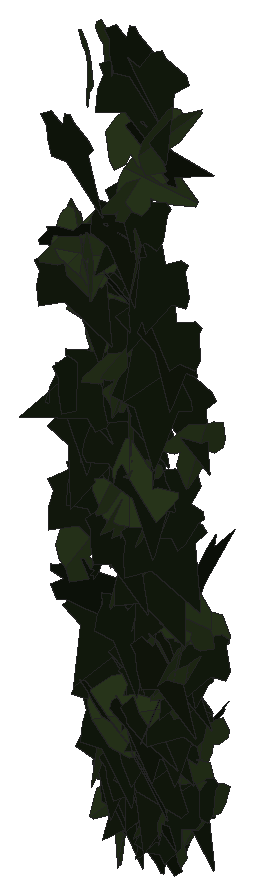
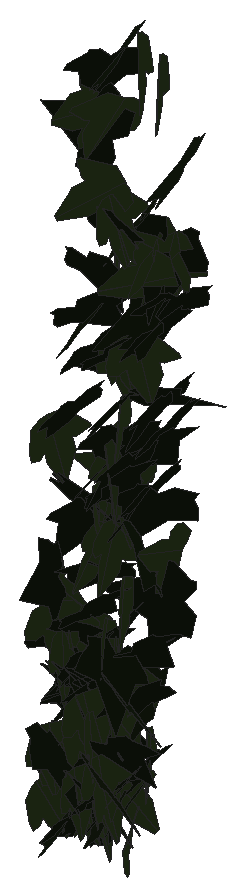
# SketchUp Ruby script. Lengths in inches.
U = 1.inch
M = Sketchup.active_model
def pt(a) = Geom::Point3d.new(a.map { |v| v * U })
def face(e, loops, mat)
  f = e.add_face(loops[0].map { |a| pt(a) })
  loops[1..].each { |l| e.add_face(l.map { |a| pt(a) }).erase! }
  f.material = f.back_material = mat if mat
  f
end
# faces: each face lists its corners as indices into pts; further lists are holes
def faces(e, pts, list, mat = nil) = list.each { |f| face(e, (f[0].is_a?(Array) ? f : [f]).map { |l| l.map { |i| pts[i] } }, mat) }
# xy, xz, yz: faces in a plane at the given z, y or x. An outline is a flat list of corners, or four numbers for a rectangle; further outlines are holes
def ring(l) = l.size == 4 ? [[l[0], l[1]], [l[2], l[1]], [l[2], l[3]], [l[0], l[3]]] : l.each_slice(2).to_a
def flat(e, list, mat, &to3) = list.each { |f| face(e, (f[0].is_a?(Array) ? f : [f]).map { |l| ring(l).map { |u, v| to3.(u, v) } }, mat) }
def xy(e, z, list, mat = nil) = flat(e, list, mat) { |x, y| [x, y, z] }
def xz(e, y, list, mat = nil) = flat(e, list, mat) { |x, z| [x, y, z] }
def yz(e, x, list, mat = nil) = flat(e, list, mat) { |y, z| [x, y, z] }
def lines(e, pts, list) = list.each { |a, b| e.add_line(pt(pts[a]), pt(pts[b])) }
# prism: a flat outline (further loops are holes) pulled along v
def prism(e, loops, v, mat = nil)
  f = face(e, loops, mat); d = Geom::Vector3d.new(v.map { |x| x * U })
  f.pushpull(f.normal.samedirection?(d) ? d.length : -d.length)
end
def box(e, o, s, mat = nil) = prism(e, [[o, [o[0] + s[0], o[1], o[2]], [o[0] + s[0], o[1] + s[1], o[2]], [o[0], o[1] + s[1], o[2]]]], [0, 0, s[2]], mat)
def at(x, y, z, deg = 0) = Geom::Transformation.translation(pt([x, y, z])) * Geom::Transformation.rotation(ORIGIN, Z_AXIS, deg.degrees)
def axes(o, x, y, z) = Geom::Transformation.new([*x, 0, *y, 0, *z, 0, *pt(o).to_a, 1])
def part(name) = M.definitions.add(name)
# library, detail: a bought-in or finely detailed component or shape, given as its bounding box
def library(name, o, s) = part(name).tap { |d| box(d.entities, o, s) }
def detail(e, o, s) = box(e.add_group.entities, o, s)
def put(e, d, t, mat = nil) = e.add_instance(d, t).tap { |i| i.material = mat if mat }
def group(e, t, mat = nil) = e.add_group.tap { |g| g.transformation = t; g.material = mat if mat }.entities
root = M.entities
M.materials.add("efeu1").color = [18, 25, 13]
M.materials.add("efeu2").color = [43, 57, 29]
c1 = part("ivyleaf_9")
p = [[1.54,2.16,1.25],[1.36,2.04,1.19],[-0.21,0.99,0.68],[-0.71,1.11,0.82],[-0.85,0.86,0.67],[-0.8,0.17,0.21],
  [-0.9,-0.01,0.1],[-0.67,-0.16,-0.02],[-0.08,-0.08,-0.05],[-0.03,-0.6,-0.4],[0.65,-0.88,-0.66],[0.83,-0.6,-0.49],
  [1.29,-0.42,-0.43],[1.8125,-0.07,-0.26],[1.21,0.44,0.15]]
faces(c1.entities,p,[[0,1,2,3,4,5,6,7,8,9,10,11,12,13,14]],"efeu1")
c2 = part("ivyleaf_10")
p = [[0,0.5,-0.03],[-0.0625,2.02,-0.43],[-0.19,2.01,-0.46],[-0.54,1.05,-0.29],[-0.52,0.625,-0.18],[-0.83,0.76,-0.28],
  [-1.16,0.64,-0.33],[-1.15,0.33,-0.24],[-0.77,-0.39,0.02],[-0.3,-0.51,0.16],[0.04,-0.48,0.23],[-0.02,2.01,-0.4375],
  [-0.06,2.01,-0.43],[0.04,-0.49,0.23],[0.67,-0.49,0.14],[1.38,0.36,-0.2],[1.375,0.51,-0.24],[0.81,0.65,-0.19],
  [0.62,0.59,-0.15],[0.6,1.09,-0.28],[0.5,1.23,-0.31]]
faces(c2.entities,p,[[0,1,2,3,4,5,6,7,8,9,10],[11,12,0,13,14,15,16,17,18,19,20]],"efeu2")
put(root,c1,axes([527.77,132.7,220.15],[0.12192,-0.89795,0.0866],[-0.00105,-0.08752,-0.9061],[0.90212,0.12126,-0.01276]))
put(root,c1,axes([527.62,132.06,228.9],[0.54732,-0.78648,0.00423],[0.00245,-0.00345,-0.95818],[0.78649,0.54733,0.00004]))
put(root,c1,axes([527.82,133.22,223.68],[0.04823,-0.91788,-0.03431],[-0.00002,0.03436,-0.91915],[0.91853,0.0482,0.00178]))
put(root,c1,axes([527.74,132.28,224.43],[0.09343,-0.78896,-0.46319],[0.1513,0.47251,-0.77432],[0.90228,0.00246,0.1778]))
put(root,c1,axes([528.55,134.35,211.66],[-0.78712,0.32185,-0.13002],[0.11038,-0.07345,-0.84998],[-0.32911,-0.7944,0.02591]))
put(root,c2,axes([528.23,131.65,215.17],[0.11401,0.3029,-0.87536],[0.19703,0.85385,0.32112],[0.90509,-0.22404,0.04036]))
put(root,c1,axes([527.62,132.2,213.89],[0.38422,0.39717,-0.69678],[0.49115,0.49428,0.55257],[0.63405,-0.62355,-0.0058]))
put(root,c2,axes([527.73,132.14,225.81],[0.51799,-0.27331,0.72979],[0.7184,-0.17212,-0.57436],[0.302,0.87823,0.11455]))
put(root,c2,axes([528.51,133.19,222.78],[-0.74652,-0.4676,0.24131],[-0.07757,-0.31648,-0.85322],[0.52044,-0.71789,0.21897]))
put(root,c1,axes([528.33,133.55,212.5],[-0.45116,-0.74076,0.1948],[-0.05928,-0.19163,-0.86601],[0.76364,-0.45252,0.04786]))
put(root,c1,axes([528.52,134.47,209.54],[-0.74101,-0.42406,-0.03234],[0.02663,0.01856,-0.85377],[0.42445,-0.74149,-0.00288]))
put(root,c1,axes([528.41,131.6,225.96],[0.60456,0.69126,-0.23101],[-0.21723,-0.1156,-0.91441],[-0.69571,0.63678,0.08478]))
put(root,c1,axes([528.66,134.03,212.42],[0.05145,0.85892,0.02038],[-0.07514,0.02483,-0.85706],[-0.85587,0.04946,0.07647]))
put(root,c1,axes([528.03,132.42,220.91],[0.37669,-0.79179,-0.36382],[-0.08597,0.36066,-0.87391],[0.86713,0.37971,0.07141]))
put(root,c2,axes([528.49,131.82,225.4375],[-0.70974,-0.61609,-0.09163],[0.0806,0.0469,-0.93968],[0.61763,-0.71409,0.01734]))
put(root,c1,axes([528.92,132.36,220.68],[-0.78747,-0.13372,0.41417],[-0.34113,-0.34209,-0.75903],[0.27028,-0.82135,0.24871]))
put(root,c1,axes([528.89,132.34,215.21],[-0.07166,0.4951,0.78388],[-0.20252,0.75888,-0.49782],[-0.90476,-0.20908,0.04934]))
put(root,c2,axes([528.66,131.77,231.76],[0.54445,-0.56301,-0.54749],[-0.10866,0.60578,-0.73101],[0.77777,0.47875,0.28113]))
put(root,c2,axes([528.63,134.52,207.98],[0.11695,-0.83454,0.06646],[0.00335,-0.06664,-0.84267],[0.83717,0.11685,-0.00591]))
put(root,c2,axes([528.61,132.4375,208.72],[0.42322,-0.68856,-0.35026],[-0.01302,0.39296,-0.78824],[0.77242,0.3839,0.17862]))
put(root,c1,axes([528.48,132.625,219.11],[-0.29439,-0.84998,0.17314],[-0.02513,-0.1744,-0.89892],[0.86707,-0.29364,0.03273]))
put(root,c1,axes([528.02,133.04,224.02],[0.83292,-0.35872,0.14303],[0.13072,-0.05806,-0.90688],[0.36339,0.84311,-0.0016]))
put(root,c1,axes([528.31,133.52,208.27],[0.01789,-0.85159,0.1942],[0.04861,-0.19296,-0.85067],[0.8721,0.02823,0.04343]))
put(root,c1,axes([529.11,134.5,208.62],[-0.68477,0.49699,0.06428],[-0.04556,0.04664,-0.84605],[-0.49906,-0.6862,-0.01095]))
put(root,c2,axes([528.54,132.4375,225.59],[-0.11036,0.85643,-0.38111],[-0.00547,-0.38432,-0.86207],[-0.93738,-0.09859,0.0499]))
put(root,c2,axes([528.8,134.52,208.63],[-0.16239,-0.84302,-0.01114],[-0.01793,0.0148,-0.85828],[0.8429,-0.1621,-0.0204]))
put(root,c2,axes([528.83,133.32,214.29],[0.2676,-0.73751,-0.40182],[0.0026,0.42245,-0.77364],[0.83987,0.23368,0.13042]))
put(root,c2,axes([528.37,131.8,225.26],[0.52823,0.39959,-0.74001],[0.56285,0.48134,0.66168],[0.62489,-0.77134,0.02955]))
put(root,c1,axes([528.42,132.31,217.32],[-0.18357,-0.70491,-0.66266],[0.31787,0.5931,-0.71897],[0.91377,-0.34793,0.11698]))
put(root,c1,axes([528.63,133.32,210.67],[-0.19432,-0.83025,-0.16051],[0.03208,0.15734,-0.85268],[0.84502,-0.1969,-0.00454]))
put(root,c2,axes([528.24,132.41,224.97],[0.24449,0.02953,0.90419],[0.63802,0.6584,-0.19403],[-0.64137,0.66622,0.15167]))
put(root,c2,axes([528.73,133.69,210.01],[0.20272,-0.66288,0.53641],[0.22648,-0.48971,-0.69076],[0.82211,0.29836,0.05803]))
put(root,c2,axes([529.36,133.05,207.27],[-0.51617,-0.33143,0.64728],[-0.54729,-0.34563,-0.61341],[0.47885,-0.7523,-0.00335]))
put(root,c1,axes([528.5,133.47,219.125],[0.33824,-0.70391,-0.45854],[-0.04899,0.47694,-0.7683],[0.83866,0.31175,0.14005]))
put(root,c1,axes([528.54,132.37,217.65],[0.25651,-0.85582,-0.15606],[-0.01895,0.15717,-0.89304],[0.86973,0.25583,0.02656]))
put(root,c2,axes([528.6,133.51,205.56],[-0.02396,-0.19022,0.85154],[0.62871,-0.59443,-0.11509],[0.60499,0.6102,0.15333]))
put(root,c2,axes([529.18,133.73,212.91],[0.22995,-0.69637,-0.47194],[-0.04496,0.47838,-0.72777],[0.84002,0.21622,0.09024]))
put(root,c1,axes([528.56,132.47,210.21],[0.69931,-0.59191,0.15775],[0.13417,-0.08559,-0.91594],[0.59769,0.71175,0.02104]))
put(root,c2,axes([529.26,134.39,209.9],[0.21597,-0.80844,-0.22185],[-0.01248,0.22596,-0.83559],[0.83823,0.21166,0.04472]))
put(root,c2,axes([529.23,133.58,218.8125],[0.40995,-0.79288,-0.14683],[0.00755,0.16849,-0.88873],[0.80633,0.40154,0.08298]))
put(root,c1,axes([528.96,134.2,207.0625],[-0.05801,-0.67643,0.53877],[0.00835,-0.5404,-0.67757],[0.86473,-0.04016,0.04269]))
put(root,c1,axes([528.76,133.3,206.92],[0.36346,-0.77962,0.17603],[0.04992,-0.17085,-0.85978],[0.79769,0.36592,-0.0264]))
put(root,c1,axes([528.81,134.24,206.89],[0.28604,-0.70731,0.40705],[0.14664,-0.37976,-0.76294],[0.80279,0.32139,-0.00567]))
put(root,c2,axes([529.38,131.85,232.3125],[0.62689,-0.55168,-0.48414],[-0.1382,0.53659,-0.79038],[0.72086,0.58263,0.2695]))
put(root,c1,axes([529.19,133.65,218.02],[-0.29528,-0.79681,0.27658],[-0.04858,-0.27649,-0.84841],[0.84205,-0.29537,0.04804]))
put(root,c1,axes([529.4,133.89,207.14],[-0.43528,-0.6341,0.34252],[-0.11311,-0.33508,-0.76407],[0.71176,-0.44104,0.08805]))
put(root,c1,axes([529.02,132.59,209.72],[0.21397,-0.90516,-0.07843],[-0.00939,0.07836,-0.93006],[0.9085,0.21399,0.00885]))
put(root,c2,axes([529.53,133.01,227.16],[-0.03887,-0.91971,0.09255],[-0.00832,-0.09228,-0.92052],[0.92432,-0.03951,-0.00439]))
put(root,c2,axes([529.59,132.52,219.9],[0.47802,-0.39709,-0.68129],[-0.1696,0.72628,-0.54231],[0.77012,0.40642,0.30346]))
put(root,c2,axes([529.49,133.04,215.85],[-0.09944,-0.77324,-0.46271],[0.07598,0.45667,-0.77947],[0.8979,-0.12427,0.01472]))
put(root,c2,axes([529.56,134.29,210.48],[-0.39789,-0.75041,0.18218],[0.01112,-0.21049,-0.84273],[0.77212,-0.38367,0.10602]))
put(root,c1,axes([529.42,133.56,222.49],[-0.41741,-0.73143,0.3281],[-0.00106,-0.36941,-0.82487],[0.80164,-0.38134,0.16975]))
put(root,c1,axes([529.16,133.05,212.94],[0.15706,-0.85192,0.05262],[0.01516,-0.05071,-0.86626],[0.85341,0.15769,0.00571]))
put(root,c1,axes([529.95,133.05,226.8],[-0.91575,-0.06933,-0.13389],[0.13276,0.01984,-0.91832],[0.07146,-0.92527,-0.00965]))
put(root,c1,axes([529.52,133.34,209.89],[-0.27953,-0.84061,-0.04696],[0.01605,0.04415,-0.88587],[0.84177,-0.27999,0.0013]))
put(root,c2,axes([529.75,132.34,217.14],[0.15934,-0.912,-0.03122],[-0.00563,0.03071,-0.92582],[0.91252,0.15944,-0.00026]))
put(root,c1,axes([529.25,132.93,220.65],[0.40228,-0.78659,-0.26275],[-0.01346,0.2858,-0.8762],[0.8292,0.38624,0.11325]))
put(root,c1,axes([529.39,132.77,219.39],[-0.19026,-0.8046,-0.46367],[0.15598,0.43889,-0.8256],[0.91545,-0.242,0.04431]))
put(root,c2,axes([529.74,133.45,206.63],[0.3539,-0.81168,-0.04704],[-0.01633,0.0442,-0.88547],[0.81288,0.35427,0.0027]))
put(root,c1,axes([529.67,133.87,211.32],[-0.36264,-0.7536,0.205],[-0.08271,-0.18769,-0.83629],[0.77659,-0.3719,0.00666]))
put(root,c1,axes([529.68,134.23,211.64],[-0.54184,-0.66738,-0.09407],[0.11451,0.02778,-0.85671],[0.66418,-0.54924,0.07097]))
put(root,c1,axes([529.59,134.04,212.375],[-0.14568,-0.86073,0.08094],[0.0013,-0.0823,-0.87285],[0.86453,-0.14492,0.01495]))
put(root,c1,axes([529.33,132.43,226.2],[0.27172,-0.86241,0.24413],[0.10161,-0.22382,-0.90375],[0.89052,0.28868,0.02863]))
put(root,c1,axes([529.42,132.04,216.4],[0.42187,-0.80198,-0.26254],[-0.12099,0.233,-0.90617],[0.83514,0.43888,0.00135]))
put(root,c2,axes([529.93,132,221.99],[-0.4002,-0.8357,0.05175],[0.01646,-0.06519,-0.92559],[0.83714,-0.39823,0.04294]))
put(root,c1,axes([529.75,134.22,213.74],[-0.34556,-0.7508,0.27495],[0.00932,-0.30329,-0.81648],[0.79951,-0.32097,0.12835]))
put(root,c2,axes([529.99,134.23,207.65],[-0.01349,-0.86483,-0.06485],[0.00995,0.0647,-0.86489],[0.8672,-0.01419,0.00892]))
put(root,c2,axes([530.01,132.9375,212.41],[-0.78204,0.35112,0.08435],[-0.07853,0.03103,-0.85723],[-0.35247,-0.78596,0.00384]))
put(root,c2,axes([529.95,132.26,222.03],[0.10795,-0.88337,0.26344],[0.06276,-0.25759,-0.88944],[0.91967,0.12127,0.02978]))
put(root,c2,axes([530,132.15,217.99],[-0.32327,-0.81143,-0.36202],[0.15563,0.32757,-0.87319],[0.87479,-0.35814,0.02157]))
put(root,c2,axes([530,133.08,215.58],[-0.01952,-0.57992,-0.6969],[0.12653,0.6885,-0.57647],[0.89775,-0.10965,0.06609]))
put(root,c2,axes([529.27,131.93,210.1],[0.31299,-0.06197,-0.93896],[0.93923,0.08135,0.30771],[0.05779,-0.98641,0.08437]))
put(root,c1,axes([530.6,132.71,206.73],[-0.54489,0.55651,0.3232],[-0.21925,0.23763,-0.7788],[-0.60505,-0.58728,-0.00886]))
put(root,c1,axes([529.6,133.63,211.05],[0.34174,-0.70724,-0.41439],[0.06098,0.46966,-0.75127],[0.81743,0.26064,0.22929]))
put(root,c2,axes([530.17,132.98,216.8],[0.35081,-0.82354,-0.15066],[-0.02596,0.15257,-0.89445],[0.83681,0.34998,0.03542]))
put(root,c1,axes([529.86,134.69,206.74],[-0.00316,-0.84491,0.07539],[0.01296,-0.07543,-0.84481],[0.84816,-0.00199,0.01319]))
put(root,c1,axes([529.68,132.45,232.33],[0.51553,-0.8013,-0.06183],[-0.03484,0.05111,-0.95281],[0.80292,0.51671,-0.00164]))
put(root,c2,axes([530.14,133.96,209.41],[-0.05704,-0.70475,0.51976],[0.1262,-0.52204,-0.69399],[0.86654,0.02964,0.13528]))
put(root,c2,axes([530.27,132.03,225.65],[0.54021,-0.71716,-0.28043],[-0.05701,0.30437,-0.8882],[0.76793,0.52709,0.13133]))
put(root,c2,axes([530.22,131.84,217.35],[0.91734,0.41204,0.03032],[-0.02797,-0.01174,1.00563],[0.41221,-0.91777,0.00075]))
put(root,c2,axes([529.78,132.82,227.74],[0.38702,0.19598,0.82773],[0.47759,0.70244,-0.38963],[-0.70388,0.58437,0.19075]))
put(root,c1,axes([530.73,132.73,205.57],[0.27196,-0.40945,0.87162],[-0.47874,0.72838,0.49153],[-0.83558,-0.55058,0.00207]))
put(root,c1,axes([530.82,134.15,211.22],[-0.84908,0.07599,0.12325],[-0.13004,-0.07772,-0.84791],[-0.06368,-0.85445,0.08809]))
put(root,c1,axes([530.38,133.67,211.26],[-0.50572,0.29814,-0.64144],[0.51179,-0.39007,-0.58481],[-0.48826,-0.71766,0.05139]))
put(root,c1,axes([529.84,132.5625,208.8],[-0.10678,-0.31698,-0.8491],[0.55658,0.65184,-0.31334],[0.71531,-0.55451,0.11705]))
put(root,c2,axes([530.98,133.08,206.2],[-0.27528,0.1691,0.78607],[-0.78077,0.14226,-0.30403],[-0.19208,-0.82064,0.10927]))
put(root,c1,axes([530.31,133.33,207.99],[-0.31895,-0.78923,-0.00888],[0.00531,0.00744,-0.85124],[0.78926,-0.31899,0.00213]))
put(root,c1,axes([529.95,133.2,214.72],[-0.03857,-0.75829,-0.43226],[0.36793,0.37823,-0.69635],[0.7915,-0.21277,0.30264]))
put(root,c1,axes([530,134.82,206.53],[0.38905,-0.74168,0.11189],[0.05313,-0.09848,-0.83753],[0.74819,0.39266,0.0013]))
put(root,c1,axes([529.9,133.01,207.93],[0.24148,-0.51982,0.65489],[0.31518,-0.57478,-0.57245],[0.77444,0.39601,0.02877]))
put(root,c1,axes([530.27,133.84,209.33],[-0.17136,-0.69715,0.48712],[0.11463,-0.51131,-0.69145],[0.84271,-0.07221,0.19311]))
put(root,c1,axes([530.62,132.86,224.99],[-0.81971,-0.29686,-0.29948],[0.28386,0.09567,-0.87178],[0.31183,-0.86744,0.00634]))
put(root,c1,axes([530.14,132.75,217.92],[0.14821,-0.86585,0.24442],[0.07881,-0.23426,-0.87767],[0.89623,0.16378,0.03676]))
put(root,c2,axes([530.25,131.96,229.98],[0.37429,0.81601,0.44998],[0.18802,0.40882,-0.89775],[-0.91269,0.41886,-0.0004]))
put(root,c1,axes([530.88,134.47,209.06],[-0.3918,0.73601,-0.2047],[0.09918,-0.1791,-0.83378],[-0.75748,-0.40414,-0.00329]))
put(root,c2,axes([530.8,133.64,208.07],[-0.548,-0.65177,0.21333],[-0.09897,-0.19506,-0.85016],[0.67862,-0.55477,0.04828]))
put(root,c1,axes([530.875,134.14,207.52],[-0.83073,-0.14055,-0.11339],[0.11143,0.02113,-0.84254],[0.14212,-0.83817,-0.00222]))
put(root,c2,axes([530.58,133.97,208.58],[0.38633,-0.74565,-0.13769],[0.09398,0.20043,-0.8217],[0.75241,0.35782,0.17334]))
put(root,c1,axes([530.09,132.45,209.88],[0.13095,-0.72975,0.60412],[0.312,-0.54262,-0.72309],[0.89451,0.29609,0.16377]))
put(root,c1,axes([530.22,133.66,211.78],[0.54761,-0.67579,-0.17608],[-0.07173,0.16815,-0.86842],[0.69466,0.55009,0.04914]))
put(root,c1,axes([531.19,133.32,217.16],[-0.85167,0.1504,0.18177],[-0.18494,-0.00282,-0.86417],[-0.14648,-0.87085,0.03419]))
put(root,c1,axes([530.28,132.69,210.37],[0.38337,-0.70979,-0.38475],[-0.06914,0.39549,-0.7985],[0.8044,0.37227,0.11473]))
put(root,c2,axes([530.76,133.87,211.99],[0.02087,-0.86574,-0.20459],[0.00053,0.20466,-0.86598],[0.88959,0.02018,0.00532]))
put(root,c1,axes([530.86,133.7,210.32],[-0.57602,-0.52426,0.42323],[-0.13202,-0.4582,-0.74726],[0.66071,-0.54862,0.21967]))
put(root,c1,axes([530.41,132.09,231.77],[-0.17482,-0.77669,-0.51982],[0.21717,0.4806,-0.79113],[0.90901,-0.2642,0.08904]))
put(root,c2,axes([530.87,134.375,208.98],[-0.32051,-0.80189,-0.0093],[0.00073,0.00973,-0.86356],[0.80194,-0.32049,-0.00293]))
put(root,c2,axes([530.72,132.93,206.99],[0.25979,-0.61321,-0.55853],[0.11663,0.60648,-0.61161],[0.82121,0.10786,0.26356]))
put(root,c1,axes([530.58,133.39,210.52],[-0.21879,-0.82495,-0.24624],[0.08866,0.23112,-0.85309],[0.85633,-0.2347,0.02541]))
put(root,c1,axes([530.46,133.79,220.48],[0.23632,-0.80397,-0.30337],[-0.02866,0.30709,-0.83613],[0.85882,0.23147,0.05557]))
put(root,c1,axes([531.48,132.55,206.88],[-0.77228,-0.07686,-0.43448],[-0.43227,-0.04373,0.7761],[-0.08843,0.88503,0.00061]))
put(root,c1,axes([531.01,132.87,223.22],[-0.58235,-0.70616,0.17703],[-0.05535,-0.1831,-0.91244],[0.7259,-0.58047,0.07245]))
put(root,c1,axes([530.6,132.74,216.33],[-0.03277,-0.66263,-0.62972],[0.12925,0.62043,-0.65959],[0.90494,-0.11262,0.0714]))
put(root,c1,axes([531.0625,133.88,214.26],[0.05157,0.32593,0.81256],[0.19666,0.78885,-0.32891],[-0.85312,0.20155,-0.0267]))
put(root,c2,axes([531.1,134.45,207],[-0.13079,-0.75175,0.3805],[-0.04244,-0.37869,-0.76276],[0.84149,-0.13594,0.02067]))
put(root,c2,axes([531.07,133.86,212.93],[-0.66937,-0.57202,0.12507],[0.06558,-0.26201,-0.84733],[0.58185,-0.62853,0.23939]))
put(root,c2,axes([531.14,132.79,212.2],[0.18523,-0.80556,-0.24121],[-0.06378,0.23282,-0.82653],[0.83848,0.19567,-0.00958]))
put(root,c1,axes([530.67,132.46,212.47],[0.51427,-0.76823,-0.21215],[-0.08987,0.19497,-0.92389],[0.7919,0.52102,0.03292]))
put(root,c1,axes([531.21,133.9,212.39],[-0.63156,-0.61459,-0.02176],[0.01524,0.01553,-0.88124],[0.61479,-0.63174,-0.0005]))
put(root,c2,axes([531.24,133.11,211.625],[-0.09506,-0.87217,-0.01301],[0.0009,0.01299,-0.87734],[0.87227,-0.09506,-0.00052]))
put(root,c2,axes([531.82,133.2,213.45],[-0.0678,-0.01497,0.88164],[-0.88041,-0.04782,-0.06852],[0.04883,-0.88295,-0.01123]))
put(root,c1,axes([530.76,133.05,222.65],[0.11529,-0.80126,0.42132],[0.10133,-0.41063,-0.80866],[0.89959,0.14894,0.0371]))
put(root,c1,axes([530.36,132.22,229.04],[0.4089,-0.27682,0.82119],[0.73422,-0.37168,-0.49088],[0.46034,0.83869,0.0535]))
put(root,c1,axes([530.92,132.22,221.69],[-0.0493,-0.92681,0.00081],[0.00233,-0.00093,-0.92812],[0.92681,-0.0493,0.00238]))
put(root,c2,axes([531.3125,133.79,219.28],[-0.28155,-0.81794,0.18961],[-0.00829,-0.19727,-0.86329],[0.83959,-0.27624,0.05506]))
put(root,c2,axes([531.17,131.78,229.63],[0.22887,-0.22668,0.96193],[-0.15545,0.96684,0.26482],[-0.97598,-0.20715,0.1834]))
